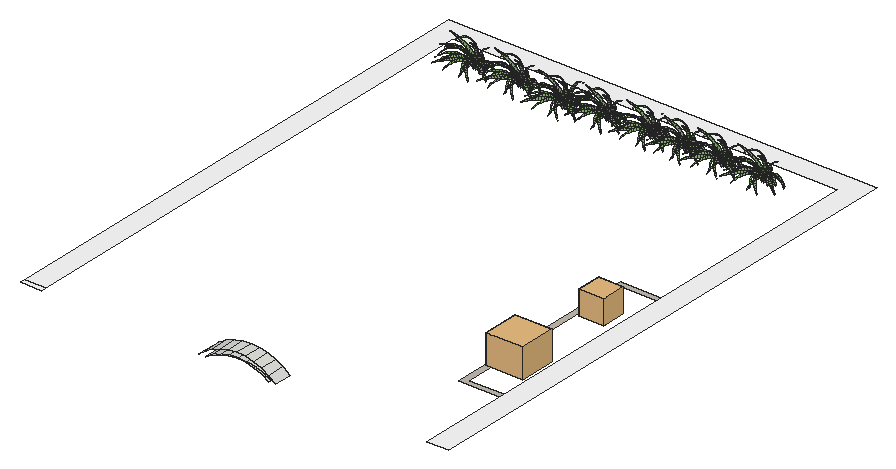
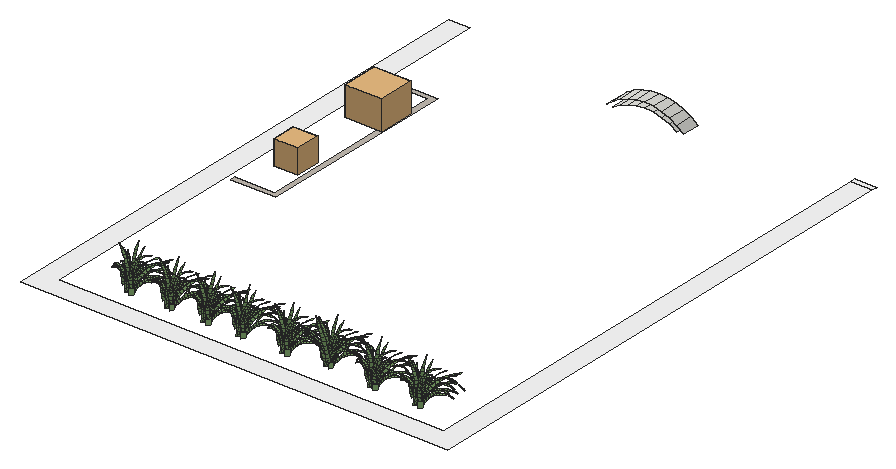
# SketchUp Ruby script. Lengths in inches.
U = 1.inch
M = Sketchup.active_model
def pt(a) = Geom::Point3d.new(a.map { |v| v * U })
def face(e, loops, mat)
  f = e.add_face(loops[0].map { |a| pt(a) })
  loops[1..].each { |l| e.add_face(l.map { |a| pt(a) }).erase! }
  f.material = f.back_material = mat if mat
  f
end
# faces: each face lists its corners as indices into pts; further lists are holes
def faces(e, pts, list, mat = nil) = list.each { |f| face(e, (f[0].is_a?(Array) ? f : [f]).map { |l| l.map { |i| pts[i] } }, mat) }
# xy, xz, yz: faces in a plane at the given z, y or x. An outline is a flat list of corners, or four numbers for a rectangle; further outlines are holes
def ring(l) = l.size == 4 ? [[l[0], l[1]], [l[2], l[1]], [l[2], l[3]], [l[0], l[3]]] : l.each_slice(2).to_a
def flat(e, list, mat, &to3) = list.each { |f| face(e, (f[0].is_a?(Array) ? f : [f]).map { |l| ring(l).map { |u, v| to3.(u, v) } }, mat) }
def xy(e, z, list, mat = nil) = flat(e, list, mat) { |x, y| [x, y, z] }
def xz(e, y, list, mat = nil) = flat(e, list, mat) { |x, z| [x, y, z] }
def yz(e, x, list, mat = nil) = flat(e, list, mat) { |y, z| [x, y, z] }
def lines(e, pts, list) = list.each { |a, b| e.add_line(pt(pts[a]), pt(pts[b])) }
# prism: a flat outline (further loops are holes) pulled along v
def prism(e, loops, v, mat = nil)
  f = face(e, loops, mat); d = Geom::Vector3d.new(v.map { |x| x * U })
  f.pushpull(f.normal.samedirection?(d) ? d.length : -d.length)
end
def box(e, o, s, mat = nil) = prism(e, [[o, [o[0] + s[0], o[1], o[2]], [o[0] + s[0], o[1] + s[1], o[2]], [o[0], o[1] + s[1], o[2]]]], [0, 0, s[2]], mat)
def at(x, y, z, deg = 0) = Geom::Transformation.translation(pt([x, y, z])) * Geom::Transformation.rotation(ORIGIN, Z_AXIS, deg.degrees)
def axes(o, x, y, z) = Geom::Transformation.new([*x, 0, *y, 0, *z, 0, *pt(o).to_a, 1])
def part(name) = M.definitions.add(name)
# library, detail: a bought-in or finely detailed component or shape, given as its bounding box
def library(name, o, s) = part(name).tap { |d| box(d.entities, o, s) }
def detail(e, o, s) = box(e.add_group.entities, o, s)
def put(e, d, t, mat = nil) = e.add_instance(d, t).tap { |i| i.material = mat if mat }
def group(e, t, mat = nil) = e.add_group.tap { |g| g.transformation = t; g.material = mat if mat }.entities
root = M.entities
M.materials.add("[Color M00]").color = [255, 255, 255]
M.materials.add("[Field Rectangle Tile]").color = [196, 189, 179]
M.materials.add("dianella").color = [131, 171, 111]
c1 = library("Group\#56",[-12.68,-11.38,-10.94],[86,86.52,68.34])
c2 = library("Group\#324",[-12.09,-12.46,-11.39],[78.97,79.26,78.14])
c3 = part("Shape Bender Component\#4")
p = [[0.27,1.78,0.46],[1.95,1.8,3.35],[1.95,4.67,3.35],[0.27,4.68,0.46],[3.06,1.81,4.8],[3.875,1.84,5.87],
  [3.875,4.64,5.87],[3.06,4.66,4.8],[6,1.9,8],[6,4.58,8],[27.35,3.23,6.09],[25.57,3.4375,7.9],
  [25.57,3.03,7.9],[23.28,2.8,9.61],[23.28,3.67,9.61],[7.08,1.93,8.8],[8.3,1.99,9.69],[8.3,4.5,9.69],
  [7.08,4.55,8.8],[23.04,2.78,9.74],[23.04,3.69,9.74],[20.86,3.86,10.86],[20.86,2.625,10.86],[10.73,2.08,10.92],
  [10.73,4.41,10.92],[12.13,2.13,11.33],[13.24,2.19,11.66],[13.24,4.3,11.66],[12.13,4.36,11.33],[18.35,2.46,11.63],
  [18.35,4.03,11.63],[15.79,2.32,11.89],[17.75,2.42,11.69],[17.75,4.07,11.69],[15.79,4.17,11.89]]
faces(c3.entities,p,[[0,1,2,3],[1,4,5,6,7,2],[5,8,9,6],[10,11,12],[13,12,11,14],[15,16,17,18,9,8],[19,13,14,20,21,22],[16,23,24,17],
  [23,25,26,27,28,24],[29,22,21,30],[31,32,29,30,33,34],[26,31,34,27]],"dianella")
c4 = part("Shape Bender Component\#5")
p = [[0.17,0.01,0.72],[1.09,0.03,4.5625],[1.09,3.73,4.5625],[0.17,3.75,0.72],[2.23,0.05,7.59],[2.48,0.0625,8.26],
  [2.48,3.71,8.26],[2.23,3.72,7.59],[4.33,0.14,11.74],[4.33,3.64,11.74],[6.2,0.2,14.41],[6.6,0.22,14.97],
  [6.6,3.56,14.97],[6.2,3.58,14.41],[9.26,0.35,17.88],[9.26,3.43,17.88],[12.27,0.4,20.43],[12.27,3.38,20.43],
  [15.58,0.51,22.59],[15.58,3.27,22.59],[19.13,0.73,24.3],[19.13,3.14,24.3],[22.875,1.08,25.56],[22.875,2.85,25.56],
  [26.75,1.47,26.33],[26.75,2.49,26.33],[30.68,1.86,26.6],[30.68,2.125,26.6],[33.95,1.875,26.45]]
faces(c4.entities,p,[[0,1,2,3],[1,4,5,6,7,2],[5,8,9,6],[8,10,11,12,13,9],[11,14,15,12],[14,16,17,15],[16,18,19,17],[18,20,21,19],
  [20,22,23,21],[22,24,25,23],[24,26,27,25],[28,27,26]],"dianella")
c5 = part("Shape Bender Component\#7")
p = [[0.01,0.94,1.17],[0.04,0.96,6.32],[0.04,4.67,6.32],[0.01,4.68,1.17],[0.42,0.98,10.52],[0.51,1,11.45],
  [0.51,4.64,11.45],[0.42,4.66,10.52],[1.4,1.07,16.52],[1.4,4.57,16.52],[2.48,1.13,20.62],[2.71,1.16,21.49],
  [2.71,4.49,21.49],[2.48,4.52,20.625],[4.4375,1.21,26.32],[4.4375,4.46,26.32],[6.56,1.22,30.98],[6.56,4.47,30.98],
  [9.06,1.29,35.43],[9.06,4.38,35.43],[11.92,1.42,39.64],[11.92,4.23,39.64],[15.13,1.74,43.57],[15.13,4,43.57],
  [18.65,2.08,47.2],[18.65,3.67,47.2],[22.46,2.47,50.5],[22.46,3.14,50.5],[25.84,2.81,52.95]]
faces(c5.entities,p,[[0,1,2,3],[1,4,5,6,7,2],[5,8,9,6],[10,11,12,13,9,8],[11,14,15,12],[14,16,17,15],[16,18,19,17],[18,20,21,19],
  [20,22,23,21],[22,24,25,23],[24,26,27,25],[28,27,26]],"dianella")
xy(root,292.1875,[[405,108.58,456,108.58,456,114.58,411,114.58,411,328.96,456,328.96,456,334.96,405,334.96]],"[Field Rectangle Tile]")
xy(root,297.0625,[[0,0,24,6],[456,0,480,0,480,600,0,600,0,6,24,6,24,576,456,576]],"[Color M00]")
p = [[196.91,24,292.04],[196.91,4,292.04],[204.3,4,297.98],[204.3,24,297.98],[204.32,6,291.98],[212.53,6,296.75],
  [212.53,4,296.75],[204.32,4,291.98],[267.6,6,296.75],[275.8,6,291.98],[275.8,4,291.98],[267.6,4,296.75],
  [275.7,24,297.98],[275.7,4,297.98],[283.09,4,292.04],[283.09,24,292.04],[204.32,24,291.98],[212.53,24,296.75],
  [267.6,24,296.75],[275.8,24,291.98],[221.35,6,300.23],[221.35,4,300.23],[258.77,6,300.23],[258.77,4,300.23],
  [221.35,24,300.23],[258.77,24,300.23],[212.49,4,302.75],[212.49,24,302.75],[267.51,24,302.75],[267.51,4,302.75],
  [230.6,6,302.35],[230.6,4,302.35],[249.52,6,302.35],[249.52,4,302.35],[230.6,24,302.35],[249.52,24,302.35],
  [240.0625,6,303.0625],[240.0625,4,303.0625],[240.0625,24,303.0625],[221.31,4,306.23],[221.31,24,306.23],[258.69,24,306.23],
  [258.69,4,306.23],[230.55,4,308.35],[230.55,24,308.35],[249.45,24,308.35],[249.45,4,308.35],[240,4,309.0625],
  [240,24,309.0625]]
faces(root,p,[[0,1,2,3],[4,5,6,7],[8,9,10,11],[12,13,14,15],[5,4,16,17],[9,8,18,19],[5,20,21,6],[22,8,11,23],
  [20,5,17,24],[8,22,25,18],[3,2,26,27],[28,29,13,12],[20,30,31,21],[32,22,23,33],[30,20,24,34],[22,32,35,25],
  [30,36,37,31],[36,32,33,37],[36,30,34,38],[32,36,38,35],[27,26,39,40],[41,42,29,28],[40,39,43,44],[45,46,42,41],
  [44,43,47,48],[48,47,46,45]])
put(root,c1,axes([441.91,150.97,297.86],[0,0.4788,0],[-0.4788,0,0],[0,0,0.4788]))
put(root,c2,axes([437.7,269.08,296.36],[0,0.34768,0],[-0.34768,0,0],[0,0,0.34768]))
put(root,c3,axes([172.27,531.45,304.42],[-0.80902,-0.55509,-0.2049],[-0.50904,0.51531,0.6897],[0.29389,-0.63549,0.63055]))
put(root,c4,axes([177.21,541.48,297.93],[-0.40056,-0.89647,-0.15707],[-0.90996,0.41292,-0.0406],[-0.10733,-0.1551,0.93042]))
put(root,c3,axes([177.62,535.63,304.47],[-0.6497,-0.75653,-0.04822],[-0.70108,0.56209,0.40231],[0.29389,-0.33158,0.85312]))
put(root,c3,axes([177.29,538.22,302.48],[-0.50805,-0.82322,-0.24691],[-0.8253,0.38347,0.37568],[0.24177,-0.42089,0.82978]))
put(root,c3,axes([178.39,541.1,306.01],[0.50638,-0.71686,-0.41224],[-0.85482,-0.38655,-0.35346],[-0.0628,-0.57888,0.77907]))
put(root,c3,axes([180.71,541.95,306.04],[0.21786,-0.91523,-0.25365],[-0.96778,-0.16344,-0.17743],[-0.12592,-0.33937,0.90275]))
put(root,c3,axes([117.78,537.45,304.42],[-0.80902,-0.55509,-0.2049],[-0.50904,0.51531,0.6897],[0.29389,-0.63549,0.63055]))
put(root,c3,axes([216.1875,537.45,304.42],[-0.80902,-0.55509,-0.2049],[-0.50904,0.51531,0.6897],[0.29389,-0.63549,0.63055]))
put(root,c3,axes([304.67,537.45,304.42],[-0.80902,-0.55509,-0.2049],[-0.50904,0.51531,0.6897],[0.29389,-0.63549,0.63055]))
put(root,c3,axes([390.87,537.45,304.42],[-0.80902,-0.55509,-0.2049],[-0.50904,0.51531,0.6897],[0.29389,-0.63549,0.63055]))
put(root,c3,axes([67.26,537.45,304.42],[-0.80902,-0.55509,-0.2049],[-0.50904,0.51531,0.6897],[0.29389,-0.63549,0.63055]))
put(root,c3,axes([265.75,537.45,304.42],[-0.80902,-0.55509,-0.2049],[-0.50904,0.51531,0.6897],[0.29389,-0.63549,0.63055]))
put(root,c3,axes([345.76,537.45,304.42],[-0.80902,-0.55509,-0.2049],[-0.50904,0.51531,0.6897],[0.29389,-0.63549,0.63055]))
put(root,c4,axes([181.2,545.01,295.62],[0.34066,-0.92115,0.08924],[-0.59285,-0.36171,-0.20421],[-0.16376,-0.01275,0.91779]))
put(root,c3,axes([180.48,542.25,300.58],[0.30902,-0.94699,0.09312],[-0.95106,-0.3077,0.03026],[0,0.08221,0.93937]))
put(root,c3,axes([176.36,537.34,308.04],[-0.70711,-0.70711,0],[-0.70408,0.70408,0.10253],[0.05813,-0.05813,0.98368]))
put(root,c3,axes([182.17,539.6875,304.7],[0.55775,-0.83001,0],[0.82646,0.55536,0.09237],[-0.06824,-0.04585,0.88619]))
put(root,c3,axes([177.34,538.07,300.03],[-0.80902,-0.58527,0.05755],[-0.50904,0.73874,0.40108],[0.29389,-0.33158,0.85312]))
put(root,c4,axes([122.72,547.48,297.93],[-0.40056,-0.89647,-0.15707],[-0.90996,0.41292,-0.0406],[-0.10733,-0.1551,0.93042]))
put(root,c4,axes([221.13,547.48,297.93],[-0.40056,-0.89647,-0.15707],[-0.90996,0.41292,-0.0406],[-0.10733,-0.1551,0.93042]))
put(root,c4,axes([309.6,547.48,297.93],[-0.40056,-0.89647,-0.15707],[-0.90996,0.41292,-0.0406],[-0.10733,-0.1551,0.93042]))
put(root,c4,axes([395.81,547.48,297.93],[-0.40056,-0.89647,-0.15707],[-0.90996,0.41292,-0.0406],[-0.10733,-0.1551,0.93042]))
put(root,c4,axes([72.2,547.48,297.93],[-0.40056,-0.89647,-0.15707],[-0.90996,0.41292,-0.0406],[-0.10733,-0.1551,0.93042]))
put(root,c4,axes([270.6875,547.48,297.93],[-0.40056,-0.89647,-0.15707],[-0.90996,0.41292,-0.0406],[-0.10733,-0.1551,0.93042]))
put(root,c4,axes([350.7,547.48,297.93],[-0.40056,-0.89647,-0.15707],[-0.90996,0.41292,-0.0406],[-0.10733,-0.1551,0.93042]))
put(root,c3,axes([123.14,541.63,304.47],[-0.6497,-0.75653,-0.04822],[-0.70108,0.56209,0.40231],[0.29389,-0.33158,0.85312]))
put(root,c3,axes([221.54,541.63,304.47],[-0.6497,-0.75653,-0.04822],[-0.70108,0.56209,0.40231],[0.29389,-0.33158,0.85312]))
put(root,c3,axes([310.02,541.63,304.47],[-0.6497,-0.75653,-0.04822],[-0.70108,0.56209,0.40231],[0.29389,-0.33158,0.85312]))
put(root,c3,axes([396.22,541.63,304.47],[-0.6497,-0.75653,-0.04822],[-0.70108,0.56209,0.40231],[0.29389,-0.33158,0.85312]))
put(root,c3,axes([72.62,541.63,304.47],[-0.6497,-0.75653,-0.04822],[-0.70108,0.56209,0.40231],[0.29389,-0.33158,0.85312]))
put(root,c3,axes([271.1,541.63,304.47],[-0.6497,-0.75653,-0.04822],[-0.70108,0.56209,0.40231],[0.29389,-0.33158,0.85312]))
put(root,c3,axes([351.11,541.63,304.47],[-0.6497,-0.75653,-0.04822],[-0.70108,0.56209,0.40231],[0.29389,-0.33158,0.85312]))
put(root,c3,axes([122.81,544.22,302.48],[-0.50805,-0.82322,-0.24691],[-0.8253,0.38347,0.37568],[0.24177,-0.42089,0.82978]))
put(root,c3,axes([221.21,544.22,302.48],[-0.50805,-0.82322,-0.24691],[-0.8253,0.38347,0.37568],[0.24177,-0.42089,0.82978]))
put(root,c3,axes([309.69,544.22,302.48],[-0.50805,-0.82322,-0.24691],[-0.8253,0.38347,0.37568],[0.24177,-0.42089,0.82978]))
put(root,c3,axes([395.9,544.22,302.48],[-0.50805,-0.82322,-0.24691],[-0.8253,0.38347,0.37568],[0.24177,-0.42089,0.82978]))
put(root,c3,axes([72.29,544.22,302.48],[-0.50805,-0.82322,-0.24691],[-0.8253,0.38347,0.37568],[0.24177,-0.42089,0.82978]))
put(root,c3,axes([270.77,544.22,302.48],[-0.50805,-0.82322,-0.24691],[-0.8253,0.38347,0.37568],[0.24177,-0.42089,0.82978]))
put(root,c3,axes([350.78,544.22,302.48],[-0.50805,-0.82322,-0.24691],[-0.8253,0.38347,0.37568],[0.24177,-0.42089,0.82978]))
put(root,c3,axes([180.59,545.99,295.75],[-0.05877,-0.98877,-0.11806],[-0.97807,0.0289,0.18451],[0.19843,-0.1475,0.9179]))
put(root,c4,axes([180.08,541.72,295.45],[-0.78227,-0.62286,0.01161],[-0.61951,0.7796,0.10187],[0.05813,-0.05813,0.98368]))
put(root,c4,axes([179.37,544.7,293.36],[0.64772,-0.76181,0.01046],[0.75801,0.64575,0.09178],[-0.06824,-0.04585,0.88619]))
put(root,c3,axes([123.9,547.1,306.01],[0.50638,-0.71686,-0.41224],[-0.85482,-0.38655,-0.35346],[-0.0628,-0.57888,0.77907]))
put(root,c3,axes([222.31,547.1,306.01],[0.50638,-0.71686,-0.41224],[-0.85482,-0.38655,-0.35346],[-0.0628,-0.57888,0.77907]))
put(root,c3,axes([310.78,547.1,306.01],[0.50638,-0.71686,-0.41224],[-0.85482,-0.38655,-0.35346],[-0.0628,-0.57888,0.77907]))
put(root,c3,axes([396.99,547.1,306.01],[0.50638,-0.71686,-0.41224],[-0.85482,-0.38655,-0.35346],[-0.0628,-0.57888,0.77907]))
put(root,c3,axes([73.38,547.1,306.01],[0.50638,-0.71686,-0.41224],[-0.85482,-0.38655,-0.35346],[-0.0628,-0.57888,0.77907]))
put(root,c3,axes([271.87,547.1,306.01],[0.50638,-0.71686,-0.41224],[-0.85482,-0.38655,-0.35346],[-0.0628,-0.57888,0.77907]))
put(root,c3,axes([351.88,547.1,306.01],[0.50638,-0.71686,-0.41224],[-0.85482,-0.38655,-0.35346],[-0.0628,-0.57888,0.77907]))
put(root,c3,axes([126.23,547.95,306.04],[0.21786,-0.91523,-0.25365],[-0.96778,-0.16344,-0.17743],[-0.12592,-0.33937,0.90275]))
put(root,c3,axes([224.64,547.95,306.04],[0.21786,-0.91523,-0.25365],[-0.96778,-0.16344,-0.17743],[-0.12592,-0.33937,0.90275]))
put(root,c3,axes([313.11,547.95,306.04],[0.21786,-0.91523,-0.25365],[-0.96778,-0.16344,-0.17743],[-0.12592,-0.33937,0.90275]))
put(root,c3,axes([399.32,547.95,306.04],[0.21786,-0.91523,-0.25365],[-0.96778,-0.16344,-0.17743],[-0.12592,-0.33937,0.90275]))
put(root,c3,axes([75.71,547.95,306.04],[0.21786,-0.91523,-0.25365],[-0.96778,-0.16344,-0.17743],[-0.12592,-0.33937,0.90275]))
put(root,c3,axes([274.2,547.95,306.04],[0.21786,-0.91523,-0.25365],[-0.96778,-0.16344,-0.17743],[-0.12592,-0.33937,0.90275]))
put(root,c3,axes([354.21,547.95,306.04],[0.21786,-0.91523,-0.25365],[-0.96778,-0.16344,-0.17743],[-0.12592,-0.33937,0.90275]))
put(root,c3,axes([182.8,543.84,300.67],[0.80902,-0.58527,0.05755],[-0.58779,-0.80556,0.07921],[0,0.08221,0.93937]))
put(root,c5,axes([179.5625,545.0625,294.24],[0.32702,-0.93868,0.09312],[-0.79728,-0.23674,0.03026],[-0.00395,0.05904,0.69543]))
put(root,c4,axes([177.44,545.74,294.5625],[0.73728,-0.6727,0.06615],[-0.67559,-0.73413,0.07219],[0,0.08221,0.93937]))
put(root,c3,axes([181.42,543.04,300.63],[0.55775,-0.83001,0],[0.78384,0.52672,-0.32887],[0.24294,0.16325,0.84049]))
put(root,c4,axes([126.72,551.01,295.62],[0.34066,-0.92115,0.08924],[-0.59285,-0.36171,-0.20421],[-0.16376,-0.01275,0.91779]))
put(root,c4,axes([225.125,551.01,295.62],[0.34066,-0.92115,0.08924],[-0.59285,-0.36171,-0.20421],[-0.16376,-0.01275,0.91779]))
put(root,c4,axes([313.6,551.01,295.62],[0.34066,-0.92115,0.08924],[-0.59285,-0.36171,-0.20421],[-0.16376,-0.01275,0.91779]))
put(root,c4,axes([399.8,551.01,295.62],[0.34066,-0.92115,0.08924],[-0.59285,-0.36171,-0.20421],[-0.16376,-0.01275,0.91779]))
put(root,c4,axes([76.2,551.01,295.62],[0.34066,-0.92115,0.08924],[-0.59285,-0.36171,-0.20421],[-0.16376,-0.01275,0.91779]))
put(root,c4,axes([274.68,551.01,295.62],[0.34066,-0.92115,0.08924],[-0.59285,-0.36171,-0.20421],[-0.16376,-0.01275,0.91779]))
put(root,c4,axes([354.69,551.01,295.62],[0.34066,-0.92115,0.08924],[-0.59285,-0.36171,-0.20421],[-0.16376,-0.01275,0.91779]))
put(root,c3,axes([176.45,551.65,294.68],[1.02343,-0.72932,-0.09719],[-1.09079,-0.98143,0.00868],[0.28212,-0.60389,1.18314]))
put(root,c3,axes([126,548.25,300.58],[0.30902,-0.94699,0.09312],[-0.95106,-0.3077,0.03026],[0,0.08221,0.93937]))
put(root,c3,axes([224.4,548.25,300.58],[0.30902,-0.94699,0.09312],[-0.95106,-0.3077,0.03026],[0,0.08221,0.93937]))
put(root,c3,axes([312.88,548.25,300.58],[0.30902,-0.94699,0.09312],[-0.95106,-0.3077,0.03026],[0,0.08221,0.93937]))
put(root,c3,axes([399.08,548.25,300.58],[0.30902,-0.94699,0.09312],[-0.95106,-0.3077,0.03026],[0,0.08221,0.93937]))
put(root,c3,axes([75.48,548.25,300.58],[0.30902,-0.94699,0.09312],[-0.95106,-0.3077,0.03026],[0,0.08221,0.93937]))
put(root,c3,axes([273.96,548.25,300.58],[0.30902,-0.94699,0.09312],[-0.95106,-0.3077,0.03026],[0,0.08221,0.93937]))
put(root,c3,axes([353.97,548.25,300.58],[0.30902,-0.94699,0.09312],[-0.95106,-0.3077,0.03026],[0,0.08221,0.93937]))
put(root,c3,axes([176.8125,539.95,295.13],[-0.80902,-0.58527,0.05755],[-0.58779,0.80556,-0.07921],[0,0.08221,0.93937]))
put(root,c3,axes([172.11,541.59,303.52],[-0.70711,-0.70711,0],[-0.66777,0.66777,-0.36504],[-0.20696,0.20696,0.93295]))
put(root,c3,axes([121.875,543.34,308.04],[-0.70711,-0.70711,0],[-0.70408,0.70408,0.10253],[0.05813,-0.05813,0.98368]))
put(root,c3,axes([220.28,543.34,308.04],[-0.70711,-0.70711,0],[-0.70408,0.70408,0.10253],[0.05813,-0.05813,0.98368]))
put(root,c3,axes([308.76,543.34,308.04],[-0.70711,-0.70711,0],[-0.70408,0.70408,0.10253],[0.05813,-0.05813,0.98368]))
put(root,c3,axes([394.96,543.34,308.04],[-0.70711,-0.70711,0],[-0.70408,0.70408,0.10253],[0.05813,-0.05813,0.98368]))
put(root,c3,axes([71.36,543.34,308.04],[-0.70711,-0.70711,0],[-0.70408,0.70408,0.10253],[0.05813,-0.05813,0.98368]))
put(root,c3,axes([269.84,543.34,308.04],[-0.70711,-0.70711,0],[-0.70408,0.70408,0.10253],[0.05813,-0.05813,0.98368]))
put(root,c3,axes([349.85,543.34,308.04],[-0.70711,-0.70711,0],[-0.70408,0.70408,0.10253],[0.05813,-0.05813,0.98368]))
put(root,c3,axes([127.69,545.6875,304.7],[0.55775,-0.83001,0],[0.82646,0.55536,0.09237],[-0.06824,-0.04585,0.88619]))
put(root,c3,axes([226.1,545.6875,304.7],[0.55775,-0.83001,0],[0.82646,0.55536,0.09237],[-0.06824,-0.04585,0.88619]))
put(root,c3,axes([314.57,545.6875,304.7],[0.55775,-0.83001,0],[0.82646,0.55536,0.09237],[-0.06824,-0.04585,0.88619]))
put(root,c3,axes([400.78,545.6875,304.7],[0.55775,-0.83001,0],[0.82646,0.55536,0.09237],[-0.06824,-0.04585,0.88619]))
put(root,c3,axes([77.17,545.6875,304.7],[0.55775,-0.83001,0],[0.82646,0.55536,0.09237],[-0.06824,-0.04585,0.88619]))
put(root,c3,axes([275.66,545.6875,304.7],[0.55775,-0.83001,0],[0.82646,0.55536,0.09237],[-0.06824,-0.04585,0.88619]))
put(root,c3,axes([355.67,545.6875,304.7],[0.55775,-0.83001,0],[0.82646,0.55536,0.09237],[-0.06824,-0.04585,0.88619]))
put(root,c3,axes([183.19,543.63,302.24],[0.91566,-0.38187,-0.12545],[-0.37002,-0.92796,0.12389],[0.1649,0.09368,0.91839]))
put(root,c3,axes([221.26,544.07,300.03],[-0.80902,-0.58527,0.05755],[-0.50904,0.73874,0.40108],[0.29389,-0.33158,0.85312]))
put(root,c3,axes([309.73,544.07,300.03],[-0.80902,-0.58527,0.05755],[-0.50904,0.73874,0.40108],[0.29389,-0.33158,0.85312]))
put(root,c3,axes([395.9375,544.07,300.03],[-0.80902,-0.58527,0.05755],[-0.50904,0.73874,0.40108],[0.29389,-0.33158,0.85312]))
put(root,c3,axes([72.33,544.07,300.03],[-0.80902,-0.58527,0.05755],[-0.50904,0.73874,0.40108],[0.29389,-0.33158,0.85312]))
put(root,c3,axes([270.82,544.07,300.03],[-0.80902,-0.58527,0.05755],[-0.50904,0.73874,0.40108],[0.29389,-0.33158,0.85312]))
put(root,c3,axes([350.83,544.07,300.03],[-0.80902,-0.58527,0.05755],[-0.50904,0.73874,0.40108],[0.29389,-0.33158,0.85312]))
put(root,c5,axes([179.12,539.09,295.59],[-0.98591,-0.15821,0.05312],[-0.14858,0.97692,0.14539],[0.05311,-0.10528,0.64334]))
put(root,c3,axes([126.11,551.99,295.75],[-0.05877,-0.98877,-0.11806],[-0.97807,0.0289,0.18451],[0.19843,-0.1475,0.9179]))
put(root,c3,axes([224.51,551.99,295.75],[-0.05877,-0.98877,-0.11806],[-0.97807,0.0289,0.18451],[0.19843,-0.1475,0.9179]))
put(root,c3,axes([312.99,551.99,295.75],[-0.05877,-0.98877,-0.11806],[-0.97807,0.0289,0.18451],[0.19843,-0.1475,0.9179]))
put(root,c3,axes([399.19,551.99,295.75],[-0.05877,-0.98877,-0.11806],[-0.97807,0.0289,0.18451],[0.19843,-0.1475,0.9179]))
put(root,c3,axes([75.59,551.99,295.75],[-0.05877,-0.98877,-0.11806],[-0.97807,0.0289,0.18451],[0.19843,-0.1475,0.9179]))
put(root,c3,axes([274.07,551.99,295.75],[-0.05877,-0.98877,-0.11806],[-0.97807,0.0289,0.18451],[0.19843,-0.1475,0.9179]))
put(root,c3,axes([354.08,551.99,295.75],[-0.05877,-0.98877,-0.11806],[-0.97807,0.0289,0.18451],[0.19843,-0.1475,0.9179]))
put(root,c5,axes([179.8,541.93,293.38],[0.93701,-0.34506,0.05429],[0.33388,0.93004,0.14862],[-0.07238,-0.09308,0.65763]))
put(root,c4,axes([125.59,547.72,295.45],[-0.78227,-0.62286,0.01161],[-0.61951,0.7796,0.10187],[0.05813,-0.05813,0.98368]))
put(root,c4,axes([224,547.72,295.45],[-0.78227,-0.62286,0.01161],[-0.61951,0.7796,0.10187],[0.05813,-0.05813,0.98368]))
put(root,c4,axes([312.47,547.72,295.45],[-0.78227,-0.62286,0.01161],[-0.61951,0.7796,0.10187],[0.05813,-0.05813,0.98368]))
put(root,c4,axes([398.68,547.72,295.45],[-0.78227,-0.62286,0.01161],[-0.61951,0.7796,0.10187],[0.05813,-0.05813,0.98368]))
put(root,c4,axes([75.07,547.72,295.45],[-0.78227,-0.62286,0.01161],[-0.61951,0.7796,0.10187],[0.05813,-0.05813,0.98368]))
put(root,c4,axes([273.56,547.72,295.45],[-0.78227,-0.62286,0.01161],[-0.61951,0.7796,0.10187],[0.05813,-0.05813,0.98368]))
put(root,c4,axes([353.57,547.72,295.45],[-0.78227,-0.62286,0.01161],[-0.61951,0.7796,0.10187],[0.05813,-0.05813,0.98368]))
put(root,c3,axes([174.37,546.49,309.08],[-0.44476,-0.68589,0.49905],[0.87828,-0.45859,0.09968],[0.1393,0.38263,0.84698]))
put(root,c4,axes([124.89,550.7,293.36],[0.64772,-0.76181,0.01046],[0.75801,0.64575,0.09178],[-0.06824,-0.04585,0.88619]))
put(root,c4,axes([223.29,550.7,293.36],[0.64772,-0.76181,0.01046],[0.75801,0.64575,0.09178],[-0.06824,-0.04585,0.88619]))
put(root,c4,axes([311.77,550.7,293.36],[0.64772,-0.76181,0.01046],[0.75801,0.64575,0.09178],[-0.06824,-0.04585,0.88619]))
put(root,c4,axes([397.97,550.7,293.36],[0.64772,-0.76181,0.01046],[0.75801,0.64575,0.09178],[-0.06824,-0.04585,0.88619]))
put(root,c4,axes([74.37,550.7,293.36],[0.64772,-0.76181,0.01046],[0.75801,0.64575,0.09178],[-0.06824,-0.04585,0.88619]))
put(root,c4,axes([272.85,550.7,293.36],[0.64772,-0.76181,0.01046],[0.75801,0.64575,0.09178],[-0.06824,-0.04585,0.88619]))
put(root,c4,axes([352.86,550.7,293.36],[0.64772,-0.76181,0.01046],[0.75801,0.64575,0.09178],[-0.06824,-0.04585,0.88619]))
put(root,c3,axes([180.45,540.45,297.625],[0.93701,-0.34506,0.05429],[0.34079,0.93717,0.07473],[-0.06824,-0.04585,0.88619]))
put(root,c3,axes([173.59,538.77,301.91],[-0.98591,-0.15821,0.06027],[-0.15399,0.98524,0.08295],[0.05813,-0.05813,0.98368]))
put(root,c3,axes([128.3125,549.84,300.67],[0.80902,-0.58527,0.05755],[-0.58779,-0.80556,0.07921],[0,0.08221,0.93937]))
put(root,c3,axes([226.72,549.84,300.67],[0.80902,-0.58527,0.05755],[-0.58779,-0.80556,0.07921],[0,0.08221,0.93937]))
put(root,c3,axes([315.19,549.84,300.67],[0.80902,-0.58527,0.05755],[-0.58779,-0.80556,0.07921],[0,0.08221,0.93937]))
put(root,c3,axes([401.4,549.84,300.67],[0.80902,-0.58527,0.05755],[-0.58779,-0.80556,0.07921],[0,0.08221,0.93937]))
put(root,c3,axes([77.79,549.84,300.67],[0.80902,-0.58527,0.05755],[-0.58779,-0.80556,0.07921],[0,0.08221,0.93937]))
put(root,c3,axes([276.28,549.84,300.67],[0.80902,-0.58527,0.05755],[-0.58779,-0.80556,0.07921],[0,0.08221,0.93937]))
put(root,c3,axes([356.29,549.84,300.67],[0.80902,-0.58527,0.05755],[-0.58779,-0.80556,0.07921],[0,0.08221,0.93937]))
put(root,c5,axes([125.08,551.0625,294.24],[0.32702,-0.93868,0.09312],[-0.79728,-0.23674,0.03026],[-0.00395,0.05904,0.69543]))
put(root,c5,axes([223.48,551.0625,294.24],[0.32702,-0.93868,0.09312],[-0.79728,-0.23674,0.03026],[-0.00395,0.05904,0.69543]))
put(root,c5,axes([311.96,551.0625,294.24],[0.32702,-0.93868,0.09312],[-0.79728,-0.23674,0.03026],[-0.00395,0.05904,0.69543]))
put(root,c5,axes([398.17,551.0625,294.24],[0.32702,-0.93868,0.09312],[-0.79728,-0.23674,0.03026],[-0.00395,0.05904,0.69543]))
put(root,c5,axes([74.56,551.0625,294.24],[0.32702,-0.93868,0.09312],[-0.79728,-0.23674,0.03026],[-0.00395,0.05904,0.69543]))
put(root,c5,axes([273.05,551.0625,294.24],[0.32702,-0.93868,0.09312],[-0.79728,-0.23674,0.03026],[-0.00395,0.05904,0.69543]))
put(root,c5,axes([353.06,551.0625,294.24],[0.32702,-0.93868,0.09312],[-0.79728,-0.23674,0.03026],[-0.00395,0.05904,0.69543]))
put(root,c4,axes([122.96,551.74,294.5625],[0.73728,-0.6727,0.06615],[-0.67559,-0.73413,0.07219],[0,0.08221,0.93937]))
put(root,c4,axes([221.36,551.74,294.5625],[0.73728,-0.6727,0.06615],[-0.67559,-0.73413,0.07219],[0,0.08221,0.93937]))
put(root,c4,axes([309.84,551.74,294.5625],[0.73728,-0.6727,0.06615],[-0.67559,-0.73413,0.07219],[0,0.08221,0.93937]))
put(root,c4,axes([396.04,551.74,294.5625],[0.73728,-0.6727,0.06615],[-0.67559,-0.73413,0.07219],[0,0.08221,0.93937]))
put(root,c4,axes([72.4375,551.74,294.5625],[0.73728,-0.6727,0.06615],[-0.67559,-0.73413,0.07219],[0,0.08221,0.93937]))
put(root,c4,axes([270.92,551.74,294.5625],[0.73728,-0.6727,0.06615],[-0.67559,-0.73413,0.07219],[0,0.08221,0.93937]))
put(root,c4,axes([350.93,551.74,294.5625],[0.73728,-0.6727,0.06615],[-0.67559,-0.73413,0.07219],[0,0.08221,0.93937]))
put(root,c3,axes([126.93,549.04,300.63],[0.55775,-0.83001,0],[0.78384,0.52672,-0.32887],[0.24294,0.16325,0.84049]))
put(root,c3,axes([225.34,549.04,300.63],[0.55775,-0.83001,0],[0.78384,0.52672,-0.32887],[0.24294,0.16325,0.84049]))
put(root,c3,axes([313.8125,549.04,300.63],[0.55775,-0.83001,0],[0.78384,0.52672,-0.32887],[0.24294,0.16325,0.84049]))
put(root,c3,axes([400.02,549.04,300.63],[0.55775,-0.83001,0],[0.78384,0.52672,-0.32887],[0.24294,0.16325,0.84049]))
put(root,c3,axes([76.41,549.04,300.63],[0.55775,-0.83001,0],[0.78384,0.52672,-0.32887],[0.24294,0.16325,0.84049]))
put(root,c3,axes([274.9,549.04,300.63],[0.55775,-0.83001,0],[0.78384,0.52672,-0.32887],[0.24294,0.16325,0.84049]))
put(root,c3,axes([354.91,549.04,300.63],[0.55775,-0.83001,0],[0.78384,0.52672,-0.32887],[0.24294,0.16325,0.84049]))
put(root,c3,axes([121.96,557.65,294.68],[1.02343,-0.72932,-0.09719],[-1.09079,-0.98143,0.00868],[0.28212,-0.60389,1.18314]))
put(root,c3,axes([220.37,557.65,294.68],[1.02343,-0.72932,-0.09719],[-1.09079,-0.98143,0.00868],[0.28212,-0.60389,1.18314]))
put(root,c3,axes([308.84,557.65,294.68],[1.02343,-0.72932,-0.09719],[-1.09079,-0.98143,0.00868],[0.28212,-0.60389,1.18314]))
put(root,c3,axes([395.05,557.65,294.68],[1.02343,-0.72932,-0.09719],[-1.09079,-0.98143,0.00868],[0.28212,-0.60389,1.18314]))
put(root,c3,axes([71.44,557.65,294.68],[1.02343,-0.72932,-0.09719],[-1.09079,-0.98143,0.00868],[0.28212,-0.60389,1.18314]))
put(root,c3,axes([269.93,557.65,294.68],[1.02343,-0.72932,-0.09719],[-1.09079,-0.98143,0.00868],[0.28212,-0.60389,1.18314]))
put(root,c3,axes([349.9375,557.65,294.68],[1.02343,-0.72932,-0.09719],[-1.09079,-0.98143,0.00868],[0.28212,-0.60389,1.18314]))
put(root,c5,axes([178.66,547.52,294.52],[0.80902,-0.58527,0.05755],[-0.58572,-0.79585,0.15754],[0.03689,0.112,0.69708]))
put(root,c3,axes([122.33,545.95,295.13],[-0.80902,-0.58527,0.05755],[-0.58779,0.80556,-0.07921],[0,0.08221,0.93937]))
put(root,c3,axes([220.73,545.95,295.13],[-0.80902,-0.58527,0.05755],[-0.58779,0.80556,-0.07921],[0,0.08221,0.93937]))
put(root,c3,axes([309.21,545.95,295.13],[-0.80902,-0.58527,0.05755],[-0.58779,0.80556,-0.07921],[0,0.08221,0.93937]))
put(root,c3,axes([395.41,545.95,295.13],[-0.80902,-0.58527,0.05755],[-0.58779,0.80556,-0.07921],[0,0.08221,0.93937]))
put(root,c3,axes([71.81,545.95,295.13],[-0.80902,-0.58527,0.05755],[-0.58779,0.80556,-0.07921],[0,0.08221,0.93937]))
put(root,c3,axes([270.29,545.95,295.13],[-0.80902,-0.58527,0.05755],[-0.58779,0.80556,-0.07921],[0,0.08221,0.93937]))
put(root,c3,axes([350.3,545.95,295.13],[-0.80902,-0.58527,0.05755],[-0.58779,0.80556,-0.07921],[0,0.08221,0.93937]))
put(root,c4,axes([180.6,543.94,293.42],[0.96956,-0.23675,0.0624],[0.23253,0.9702,0.0681],[-0.06824,-0.04585,0.88619]))
put(root,c3,axes([117.625,547.59,303.52],[-0.70711,-0.70711,0],[-0.66777,0.66777,-0.36504],[-0.20696,0.20696,0.93295]))
put(root,c3,axes([216.03,547.59,303.52],[-0.70711,-0.70711,0],[-0.66777,0.66777,-0.36504],[-0.20696,0.20696,0.93295]))
put(root,c3,axes([304.51,547.59,303.52],[-0.70711,-0.70711,0],[-0.66777,0.66777,-0.36504],[-0.20696,0.20696,0.93295]))
put(root,c3,axes([390.71,547.59,303.52],[-0.70711,-0.70711,0],[-0.66777,0.66777,-0.36504],[-0.20696,0.20696,0.93295]))
put(root,c3,axes([67.1,547.59,303.52],[-0.70711,-0.70711,0],[-0.66777,0.66777,-0.36504],[-0.20696,0.20696,0.93295]))
put(root,c3,axes([265.59,547.59,303.52],[-0.70711,-0.70711,0],[-0.66777,0.66777,-0.36504],[-0.20696,0.20696,0.93295]))
put(root,c3,axes([345.6,547.59,303.52],[-0.70711,-0.70711,0],[-0.66777,0.66777,-0.36504],[-0.20696,0.20696,0.93295]))
put(root,c4,axes([178.72,541.22,295.51],[-0.99701,-0.04566,0.06927],[-0.04139,0.99682,0.07559],[0.05813,-0.05813,0.98368]))
put(root,c3,axes([128.71,549.63,302.24],[0.91566,-0.38187,-0.12545],[-0.37002,-0.92796,0.12389],[0.1649,0.09368,0.91839]))
put(root,c3,axes([227.11,549.63,302.24],[0.91566,-0.38187,-0.12545],[-0.37002,-0.92796,0.12389],[0.1649,0.09368,0.91839]))
put(root,c3,axes([315.59,549.63,302.24],[0.91566,-0.38187,-0.12545],[-0.37002,-0.92796,0.12389],[0.1649,0.09368,0.91839]))
put(root,c3,axes([401.79,549.63,302.24],[0.91566,-0.38187,-0.12545],[-0.37002,-0.92796,0.12389],[0.1649,0.09368,0.91839]))
put(root,c3,axes([78.1875,549.63,302.24],[0.91566,-0.38187,-0.12545],[-0.37002,-0.92796,0.12389],[0.1649,0.09368,0.91839]))
put(root,c3,axes([276.67,549.63,302.24],[0.91566,-0.38187,-0.12545],[-0.37002,-0.92796,0.12389],[0.1649,0.09368,0.91839]))
put(root,c3,axes([356.68,549.63,302.24],[0.91566,-0.38187,-0.12545],[-0.37002,-0.92796,0.12389],[0.1649,0.09368,0.91839]))
put(root,c5,axes([124.64,545.09,295.59],[-0.98591,-0.15821,0.05312],[-0.14858,0.97692,0.14539],[0.05311,-0.10528,0.64334]))
put(root,c5,axes([223.04,545.09,295.59],[-0.98591,-0.15821,0.05312],[-0.14858,0.97692,0.14539],[0.05311,-0.10528,0.64334]))
put(root,c5,axes([311.52,545.09,295.59],[-0.98591,-0.15821,0.05312],[-0.14858,0.97692,0.14539],[0.05311,-0.10528,0.64334]))
put(root,c5,axes([397.72,545.09,295.59],[-0.98591,-0.15821,0.05312],[-0.14858,0.97692,0.14539],[0.05311,-0.10528,0.64334]))
put(root,c5,axes([74.12,545.09,295.59],[-0.98591,-0.15821,0.05312],[-0.14858,0.97692,0.14539],[0.05311,-0.10528,0.64334]))
put(root,c5,axes([272.6,545.09,295.59],[-0.98591,-0.15821,0.05312],[-0.14858,0.97692,0.14539],[0.05311,-0.10528,0.64334]))
put(root,c5,axes([352.61,545.09,295.59],[-0.98591,-0.15821,0.05312],[-0.14858,0.97692,0.14539],[0.05311,-0.10528,0.64334]))
put(root,c5,axes([125.32,547.93,293.38],[0.93701,-0.34506,0.05429],[0.33388,0.93004,0.14862],[-0.07238,-0.09308,0.65763]))
put(root,c5,axes([223.72,547.93,293.38],[0.93701,-0.34506,0.05429],[0.33388,0.93004,0.14862],[-0.07238,-0.09308,0.65763]))
put(root,c5,axes([312.2,547.93,293.38],[0.93701,-0.34506,0.05429],[0.33388,0.93004,0.14862],[-0.07238,-0.09308,0.65763]))
put(root,c5,axes([398.4,547.93,293.38],[0.93701,-0.34506,0.05429],[0.33388,0.93004,0.14862],[-0.07238,-0.09308,0.65763]))
put(root,c5,axes([74.8,547.93,293.38],[0.93701,-0.34506,0.05429],[0.33388,0.93004,0.14862],[-0.07238,-0.09308,0.65763]))
put(root,c5,axes([273.28,547.93,293.38],[0.93701,-0.34506,0.05429],[0.33388,0.93004,0.14862],[-0.07238,-0.09308,0.65763]))
put(root,c5,axes([353.29,547.93,293.38],[0.93701,-0.34506,0.05429],[0.33388,0.93004,0.14862],[-0.07238,-0.09308,0.65763]))
put(root,c4,axes([176.125,546.34,294.5],[0.99357,-0.11272,0.01108],[-0.1132,-0.98932,0.09728],[0,0.08221,0.93937]))
put(root,c3,axes([119.88,552.49,309.08],[-0.44476,-0.68589,0.49905],[0.87828,-0.45859,0.09968],[0.1393,0.38263,0.84698]))
put(root,c3,axes([218.29,552.49,309.08],[-0.44476,-0.68589,0.49905],[0.87828,-0.45859,0.09968],[0.1393,0.38263,0.84698]))
put(root,c3,axes([306.76,552.49,309.08],[-0.44476,-0.68589,0.49905],[0.87828,-0.45859,0.09968],[0.1393,0.38263,0.84698]))
put(root,c3,axes([392.97,552.49,309.08],[-0.44476,-0.68589,0.49905],[0.87828,-0.45859,0.09968],[0.1393,0.38263,0.84698]))
put(root,c3,axes([69.36,552.49,309.08],[-0.44476,-0.68589,0.49905],[0.87828,-0.45859,0.09968],[0.1393,0.38263,0.84698]))
put(root,c3,axes([267.85,552.49,309.08],[-0.44476,-0.68589,0.49905],[0.87828,-0.45859,0.09968],[0.1393,0.38263,0.84698]))
put(root,c3,axes([347.86,552.49,309.08],[-0.44476,-0.68589,0.49905],[0.87828,-0.45859,0.09968],[0.1393,0.38263,0.84698]))
put(root,c3,axes([181.85,546.81,306.52],[1,0,0],[0,-0.99572,0.09791],[0,0.08221,0.93937]))
put(root,c3,axes([125.96,546.45,297.625],[0.93701,-0.34506,0.05429],[0.34079,0.93717,0.07473],[-0.06824,-0.04585,0.88619]))
put(root,c3,axes([224.37,546.45,297.625],[0.93701,-0.34506,0.05429],[0.34079,0.93717,0.07473],[-0.06824,-0.04585,0.88619]))
put(root,c3,axes([312.84,546.45,297.625],[0.93701,-0.34506,0.05429],[0.34079,0.93717,0.07473],[-0.06824,-0.04585,0.88619]))
put(root,c3,axes([399.05,546.45,297.625],[0.93701,-0.34506,0.05429],[0.34079,0.93717,0.07473],[-0.06824,-0.04585,0.88619]))
put(root,c3,axes([75.44,546.45,297.625],[0.93701,-0.34506,0.05429],[0.34079,0.93717,0.07473],[-0.06824,-0.04585,0.88619]))
put(root,c3,axes([273.93,546.45,297.625],[0.93701,-0.34506,0.05429],[0.34079,0.93717,0.07473],[-0.06824,-0.04585,0.88619]))
put(root,c3,axes([353.9375,546.45,297.625],[0.93701,-0.34506,0.05429],[0.34079,0.93717,0.07473],[-0.06824,-0.04585,0.88619]))
put(root,c3,axes([119.11,544.77,301.91],[-0.98591,-0.15821,0.06027],[-0.15399,0.98524,0.08295],[0.05813,-0.05813,0.98368]))
put(root,c3,axes([217.51,544.77,301.91],[-0.98591,-0.15821,0.06027],[-0.15399,0.98524,0.08295],[0.05813,-0.05813,0.98368]))
put(root,c3,axes([305.99,544.77,301.91],[-0.98591,-0.15821,0.06027],[-0.15399,0.98524,0.08295],[0.05813,-0.05813,0.98368]))
put(root,c3,axes([392.19,544.77,301.91],[-0.98591,-0.15821,0.06027],[-0.15399,0.98524,0.08295],[0.05813,-0.05813,0.98368]))
put(root,c3,axes([68.59,544.77,301.91],[-0.98591,-0.15821,0.06027],[-0.15399,0.98524,0.08295],[0.05813,-0.05813,0.98368]))
